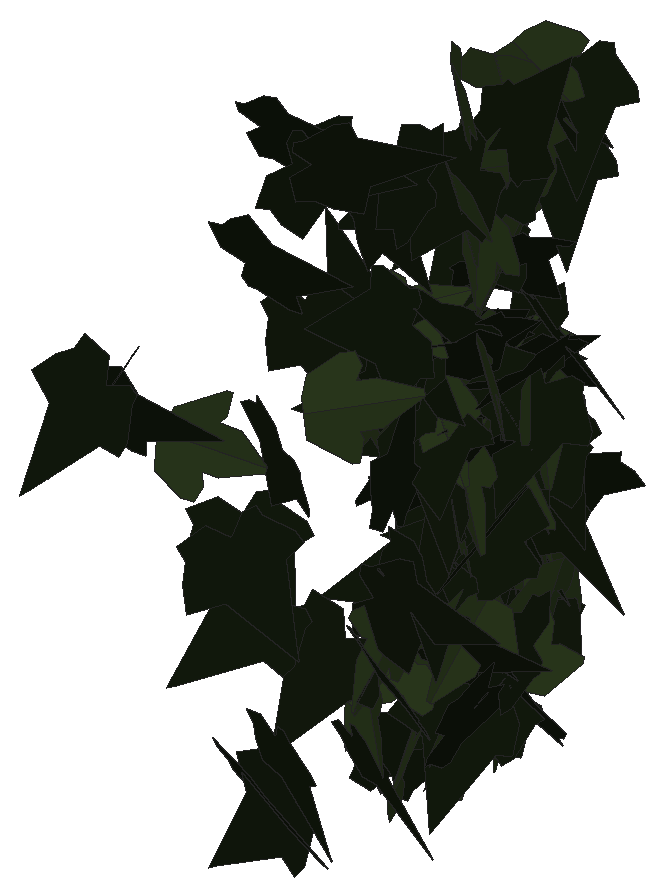
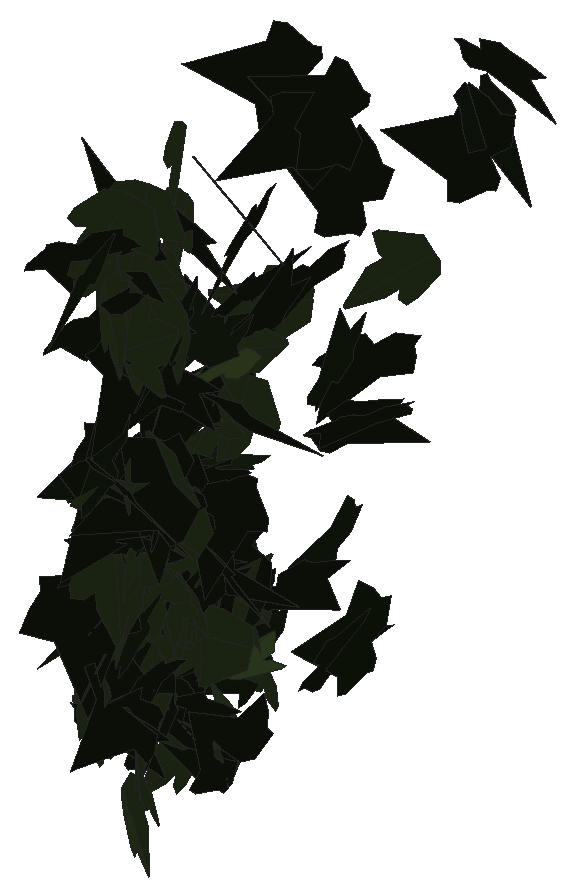
# SketchUp Ruby script. Lengths in inches.
U = 1.inch
M = Sketchup.active_model
def pt(a) = Geom::Point3d.new(a.map { |v| v * U })
def face(e, loops, mat)
  f = e.add_face(loops[0].map { |a| pt(a) })
  loops[1..].each { |l| e.add_face(l.map { |a| pt(a) }).erase! }
  f.material = f.back_material = mat if mat
  f
end
# faces: each face lists its corners as indices into pts; further lists are holes
def faces(e, pts, list, mat = nil) = list.each { |f| face(e, (f[0].is_a?(Array) ? f : [f]).map { |l| l.map { |i| pts[i] } }, mat) }
# xy, xz, yz: faces in a plane at the given z, y or x. An outline is a flat list of corners, or four numbers for a rectangle; further outlines are holes
def ring(l) = l.size == 4 ? [[l[0], l[1]], [l[2], l[1]], [l[2], l[3]], [l[0], l[3]]] : l.each_slice(2).to_a
def flat(e, list, mat, &to3) = list.each { |f| face(e, (f[0].is_a?(Array) ? f : [f]).map { |l| ring(l).map { |u, v| to3.(u, v) } }, mat) }
def xy(e, z, list, mat = nil) = flat(e, list, mat) { |x, y| [x, y, z] }
def xz(e, y, list, mat = nil) = flat(e, list, mat) { |x, z| [x, y, z] }
def yz(e, x, list, mat = nil) = flat(e, list, mat) { |y, z| [x, y, z] }
def lines(e, pts, list) = list.each { |a, b| e.add_line(pt(pts[a]), pt(pts[b])) }
# prism: a flat outline (further loops are holes) pulled along v
def prism(e, loops, v, mat = nil)
  f = face(e, loops, mat); d = Geom::Vector3d.new(v.map { |x| x * U })
  f.pushpull(f.normal.samedirection?(d) ? d.length : -d.length)
end
def box(e, o, s, mat = nil) = prism(e, [[o, [o[0] + s[0], o[1], o[2]], [o[0] + s[0], o[1] + s[1], o[2]], [o[0], o[1] + s[1], o[2]]]], [0, 0, s[2]], mat)
def at(x, y, z, deg = 0) = Geom::Transformation.translation(pt([x, y, z])) * Geom::Transformation.rotation(ORIGIN, Z_AXIS, deg.degrees)
def axes(o, x, y, z) = Geom::Transformation.new([*x, 0, *y, 0, *z, 0, *pt(o).to_a, 1])
def part(name) = M.definitions.add(name)
# library, detail: a bought-in or finely detailed component or shape, given as its bounding box
def library(name, o, s) = part(name).tap { |d| box(d.entities, o, s) }
def detail(e, o, s) = box(e.add_group.entities, o, s)
def put(e, d, t, mat = nil) = e.add_instance(d, t).tap { |i| i.material = mat if mat }
def group(e, t, mat = nil) = e.add_group.tap { |g| g.transformation = t; g.material = mat if mat }.entities
root = M.entities
M.materials.add("efeu1").color = [18, 25, 13]
M.materials.add("efeu2").color = [43, 57, 29]
c1 = part("ivyleaf_9")
p = [[1.54,2.16,1.25],[1.36,2.04,1.19],[-0.21,0.99,0.68],[-0.71,1.11,0.82],[-0.85,0.86,0.67],[-0.8,0.17,0.21],
  [-0.9,-0.01,0.1],[-0.67,-0.16,-0.02],[-0.08,-0.08,-0.05],[-0.03,-0.6,-0.4],[0.65,-0.88,-0.66],[0.83,-0.6,-0.49],
  [1.29,-0.42,-0.43],[1.8125,-0.07,-0.26],[1.21,0.44,0.15]]
faces(c1.entities,p,[[0,1,2,3,4,5,6,7,8,9,10,11,12,13,14]],"efeu1")
c2 = part("ivyleaf_10")
p = [[0,0.5,-0.03],[-0.0625,2.02,-0.43],[-0.19,2.01,-0.46],[-0.54,1.05,-0.29],[-0.52,0.625,-0.18],[-0.83,0.76,-0.28],
  [-1.16,0.64,-0.33],[-1.15,0.33,-0.24],[-0.77,-0.39,0.02],[-0.3,-0.51,0.16],[0.04,-0.48,0.23],[-0.02,2.01,-0.4375],
  [-0.06,2.01,-0.43],[0.04,-0.49,0.23],[0.67,-0.49,0.14],[1.38,0.36,-0.2],[1.375,0.51,-0.24],[0.81,0.65,-0.19],
  [0.62,0.59,-0.15],[0.6,1.09,-0.28],[0.5,1.23,-0.31]]
faces(c2.entities,p,[[0,1,2,3,4,5,6,7,8,9,10],[11,12,0,13,14,15,16,17,18,19,20]],"efeu2")
put(root,c1,axes([52.54,222,233.4],[-0.12743,-0.13778,0.46344],[0.30064,0.35276,0.18755],[-0.37865,0.32646,-0.00706]))
put(root,c1,axes([52.47,223.08,240.19],[0.37005,-0.22634,-0.24867],[-0.21472,0.1255,-0.43376],[0.25877,0.42781,-0.00432]))
put(root,c1,axes([52.57,223.91,235.06],[0.14272,0.35572,0.32109],[0.12597,0.29539,-0.38324],[-0.46234,0.19029,-0.0053]))
put(root,c1,axes([52.22,219.8,234.22],[0.374,-0.25873,0.2078],[0.17217,-0.11637,-0.45477],[0.28369,0.41173,0.00205]))
put(root,c1,axes([52.32,219.75,237.35],[0.0377,-0.46985,-0.16678],[0.17017,0.16934,-0.4386],[0.46864,-0.02369,0.17268]))
put(root,c1,axes([52.33,223.42,237.99],[0.39492,0.17488,0.25191],[0.21611,0.1327,-0.43091],[-0.21757,0.44923,0.02923]))
put(root,c2,axes([52.91,223.47,239.78],[-0.23646,0.11889,-0.42421],[-0.36386,0.21873,0.26412],[0.24838,0.43361,-0.01693]))
put(root,c1,axes([52.625,221.02,235.4],[-0.25003,-0.4141,0.12651],[-0.06772,-0.10689,-0.48372],[0.42767,-0.25902,-0.00264]))
put(root,c2,axes([52.43,223.35,240.21],[-0.3398,0.20353,-0.30514],[0.24386,-0.18535,-0.39519],[-0.27399,-0.4174,0.0267]))
put(root,c1,axes([53,221.84,238.15],[-0.4116,0.12746,0.25365],[-0.26788,-0.02654,-0.42135],[-0.09394,-0.48275,0.09013]))
put(root,c2,axes([52.63,222.03,234.64],[-0.47623,-0.02563,0.15016],[0.06941,-0.47525,0.13899],[0.1356,0.15323,0.45622]))
put(root,c1,axes([52.21,220.25,241.83],[0.28379,0.17344,-0.37334],[0.32837,0.1781,0.33235],[0.24827,-0.43382,-0.01282]))
put(root,c2,axes([52.64,223.34,234.63],[-0.09644,0.44196,0.213],[-0.07762,0.2006,-0.45137],[-0.48443,-0.12013,0.02992]))
put(root,c2,axes([52.62,223.97,233.59],[0.22192,-0.44085,0.08005],[0.04515,-0.06687,-0.49345],[0.44577,0.22624,0.01013]))
put(root,c1,axes([52.82,216.8,240.35],[-0.28664,0.37913,-0.15524],[0.09516,-0.12267,-0.47529],[-0.39847,-0.30202,-0.00183]))
put(root,c1,axes([52.75,223.39,239.44],[-0.45151,-0.2066,-0.05876],[0.06151,0.00669,-0.49616],[0.2058,-0.45527,0.01937]))
put(root,c1,axes([52.73,221.97,237.1875],[0.1117,0.48678,0.02385],[0.00703,0.02286,-0.49943],[-0.48731,0.11191,-0.00174]))
put(root,c2,axes([52.51,223.09,236.35],[0.4207,-0.21305,0.16621],[0.15861,-0.05428,-0.47106],[0.21876,0.44907,0.02191]))
put(root,c2,axes([52.79,223.36,236.97],[0.07256,0.12483,0.4787],[-0.25109,0.42616,-0.07307],[-0.42625,-0.22979,0.12453]))
put(root,c1,axes([52.83,223.27,237.96],[-0.03612,0.49855,0.01178],[-0.00711,0.01129,-0.49982],[-0.49864,-0.03628,0.00627]))
put(root,c2,axes([52.38,223.24,237.09],[-0.20906,-0.1301,0.43517],[0.37201,0.22579,0.24622],[-0.26058,0.42672,0.00239]))
put(root,c1,axes([52.6875,220.09,233.875],[-0.14326,-0.29748,0.37548],[-0.13764,-0.34982,-0.32967],[0.45884,-0.19782,0.01834]))
put(root,c1,axes([52.8125,221.21,239.09],[-0.15478,-0.41276,0.23595],[0.10415,0.21268,0.44036],[-0.46389,0.18547,0.02014]))
put(root,c1,axes([52.47,220.1875,238.04],[-0.00705,-0.27387,0.41827],[0.11007,-0.40889,-0.26588],[0.48768,0.08833,0.06605]))
put(root,c2,axes([52.51,218.49,238.91],[0.08143,0.20329,0.44949],[0.16024,0.41997,-0.21897],[-0.46658,0.17971,0.00324]))
put(root,c2,axes([52.91,223.1,236.1],[-0.45999,0.01901,0.19505],[-0.19532,-0.08516,-0.45233],[0.01602,-0.49233,0.08577]))
put(root,c2,axes([52.36,223.39,238.02],[0.26856,0.00029,0.42175],[0.42173,0.00518,-0.26855],[-0.00452,0.49997,0.00254]))
put(root,c2,axes([52.88,221.66,233.48],[0.1955,-0.08855,0.4516],[-0.28684,0.36024,0.19481],[-0.35987,-0.33524,0.09006]))
put(root,c2,axes([52.52,223.88,234.04],[0.3234,-0.23048,0.30379],[0.26475,-0.15097,-0.39638],[0.27444,0.41724,0.0244]))
put(root,c1,axes([52.5625,220.53,239.68],[0.13999,-0.42507,-0.22297],[-0.04554,0.21945,-0.44695],[0.47784,0.14545,0.02273]))
put(root,c2,axes([52.77,222.9,235.9],[-0.41577,0.27742,0.01329],[-0.01509,0.00132,-0.49977],[-0.27733,-0.41598,0.00728]))
put(root,c2,axes([52.61,221.97,239.01],[0.43239,-0.13329,-0.21278],[0.16186,0.4719,0.0333],[0.19195,-0.09768,0.45124]))
put(root,c2,axes([52.875,223.98,236.92],[-0.38979,-0.30826,0.05513],[-0.04397,-0.03327,-0.49695],[0.31005,-0.39226,-0.00118]))
put(root,c1,axes([52.99,222.25,236.43],[-0.49114,0.08693,-0.03502],[0.03433,-0.00701,-0.49877],[-0.08721,-0.49233,0.00092]))
put(root,c1,axes([52.35,219.81,240.44],[0.18372,-0.12807,0.44704],[0.40533,-0.1915,-0.22144],[0.22794,0.44376,0.03345]))
put(root,c2,axes([52.42,222.25,235.1875],[0.11033,-0.00862,-0.4876],[0.46689,0.14627,0.10306],[0.14087,-0.47805,0.04032]))
put(root,c2,axes([52.83,221.66,238.97],[-0.09962,0.18434,-0.45398],[-0.13483,-0.45569,-0.15545],[-0.47106,0.09145,0.1405]))
put(root,c1,axes([52.84,222.84,235.66],[-0.11595,-0.21492,0.43631],[-0.21428,-0.38009,-0.24417],[0.43662,-0.24361,-0.00396]))
put(root,c1,axes([53.12,222.23,236.02],[-0.42038,-0.04415,0.26707],[-0.26448,-0.03811,-0.42261],[0.05767,-0.49659,0.00869]))
put(root,c1,axes([52.66,223.93,235.15],[-0.03109,-0.49497,0.06354],[-0.01283,-0.06285,-0.49587],[0.49887,-0.03246,-0.00879]))
put(root,c1,axes([53.125,223.87,238],[-0.45371,0.17036,0.123],[-0.1198,0.03073,-0.48446],[-0.17262,-0.46908,0.01293]))
put(root,c2,axes([52.86,223.42,238.02],[0.0425,-0.49817,-0.00431],[-0.00458,0.00394,-0.49996],[0.49817,0.04254,-0.00422]))
put(root,c1,axes([52.6,223.73,236.08],[0.38289,-0.31099,-0.08171],[-0.06145,0.05394,-0.49327],[0.31562,0.38778,0.00309]))
put(root,c2,axes([52.84,221.46,238.21],[-0.09418,-0.41566,-0.26146],[0.06945,0.25227,-0.42607],[0.48611,-0.11657,0.01022]))
put(root,c1,axes([52.57,222.9,237.42],[0.37894,0.12388,0.30176],[0.24718,0.19277,-0.38954],[-0.21285,0.44441,0.08485]))
put(root,c2,axes([52.68,222.33,235.25],[0.018,-0.17464,-0.46816],[0.2738,0.39532,-0.13695],[0.41798,-0.25143,0.10986]))
put(root,c1,axes([52.76,221.38,240.76],[0.27369,-0.27786,-0.31287],[-0.21444,0.22789,-0.38997],[0.35932,0.34765,0.00557]))
put(root,c1,axes([52.7,220.19,241.58],[0.07228,0.06448,-0.49053],[-0.03702,0.49505,0.05962],[0.49336,0.0277,0.07634]))
put(root,c1,axes([52.4375,217.19,239.88],[0.28667,-0.06983,0.40366],[0.3897,-0.10543,-0.29499],[0.12631,0.48374,-0.00602]))
put(root,c2,axes([52.79,223.56,236.57],[0.4657,0.18166,-0.01117],[-0.00989,-0.00538,-0.49987],[-0.18174,0.4658,-0.00142]))
put(root,c1,axes([52.79,223.39,237.56],[0.42579,-0.08179,-0.24902],[-0.23767,0.07984,-0.4326],[0.11052,0.48676,0.02911]))
put(root,c2,axes([53.03,222.99,236.19],[-0.2906,-0.32651,0.24279],[-0.11953,-0.21668,-0.43447],[0.38893,-0.31055,0.04788]))
put(root,c2,axes([52.6,221.42,234.52],[0.30034,-0.14463,0.37266],[0.35553,-0.11644,-0.33172],[0.18274,0.46424,0.0329]))
put(root,c2,axes([52.93,223.89,235.47],[-0.07918,0.49287,0.02846],[-0.08407,0.01494,-0.49266],[-0.48648,-0.08281,0.0805]))
put(root,c2,axes([52.79,223.78,237.8125],[0.24713,0.40604,0.1551],[0.0681,0.14004,-0.47513],[-0.42929,0.25597,0.01391]))
put(root,c2,axes([52.87,221.61,235.4],[-0.04538,-0.30078,0.39682],[0.14398,-0.38937,-0.27867],[0.47667,0.08898,0.12195]))
put(root,c1,axes([53.08,219.3,236.78],[-0.34226,-0.2941,0.21533],[-0.15663,-0.14805,-0.45116],[0.32913,-0.37628,0.00921]))
put(root,c1,axes([52.86,221.6,238.81],[0.16506,-0.21205,-0.42165],[-0.20934,0.36746,-0.26674],[0.423,0.26459,0.03253]))
put(root,c1,axes([52.92,223.95,237.06],[-0.3232,-0.37439,-0.07332],[0.05656,0.04801,-0.49447],[0.37728,-0.32792,0.01131]))
put(root,c1,axes([53.04,223.97,234.71],[-0.45814,-0.18174,-0.08415],[0.08637,0.01028,-0.49238],[0.1807,-0.46569,0.02198]))
put(root,c2,axes([53.15,224.19,235.08],[0.25927,-0.11087,-0.4129],[-0.25229,0.35017,-0.25244],[0.34515,0.33924,0.12564]))
put(root,c1,axes([52.81,223.5,236.59],[0.39833,-0.2769,-0.12106],[0.09584,-0.0742,0.48509],[-0.28661,-0.40966,-0.00603]))
put(root,c1,axes([53.13,216.33,240.72],[-0.48736,-0.09764,-0.05426],[0.05338,0.00979,-0.49705],[0.09813,-0.49028,0.00088]))
put(root,c2,axes([52.93,223.8,236.14],[-0.34201,0.34766,-0.11026],[0.06761,-0.0881,-0.48751],[-0.35841,-0.34838,0.01325]))
put(root,c1,axes([52.93,223.62,237.78],[0.2958,0.37907,0.13715],[0.065,0.12303,-0.48025],[-0.39784,0.30194,0.0235]))
put(root,c1,axes([52.68,223.44,234.32],[0.11825,-0.25127,0.41579],[0.19304,-0.3684,-0.27753],[0.44582,0.22616,0.00988]))
put(root,c2,axes([53.19,222.47,235.54],[-0.15909,-0.25945,0.39671],[-0.16932,-0.35974,-0.30318],[0.44274,-0.23081,0.0266]))
put(root,c2,axes([52.97,222.95,235.46],[-0.20052,0.4577,-0.01735],[0.00964,-0.01472,-0.49969],[-0.45793,-0.20074,-0.00292]))
put(root,c2,axes([53.04,222.32,233.63],[0.05784,0.11816,0.48238],[-0.12938,0.47246,-0.10022],[-0.47949,-0.11323,0.08523]))
put(root,c1,axes([52.91,222.46,237.37],[-0.08067,-0.48674,-0.08109],[0.03533,0.07626,-0.49289],[0.49218,-0.08525,0.02209]))
put(root,c1,axes([53.17,222.26,237.14],[0.052,0.4968,-0.02213],[-0.00281,-0.02196,-0.49951],[-0.49728,0.05208,0.00051]))
put(root,c2,axes([52.85,222.26,237.93],[-0.12365,-0.48419,0.01654],[0.34608,-0.10022,-0.34668],[0.33903,-0.07429,0.35991]))
put(root,c1,axes([53.29,222.9375,240.0625],[-0.48694,0.10081,-0.05224],[-0.05099,0.01138,0.49726],[0.10144,0.4896,-0.0008]))
put(root,c2,axes([53.11,223.15,241.57],[-0.49374,-0.07449,-0.02586],[0.02587,0.00188,-0.49933],[0.07448,-0.49442,0.002]))
put(root,c1,axes([52.81,222.25,237.61],[-0.12369,-0.48261,-0.04229],[0.34495,-0.05709,-0.35743],[0.34017,-0.11759,0.34707]))
put(root,c1,axes([53.38,222.97,234.1875],[-0.45839,-0.06228,0.18973],[-0.18551,-0.04299,-0.46232],[0.0739,-0.49424,0.01631]))
put(root,c1,axes([53.4,221.43,241.1],[-0.43341,0.23508,0.08301],[-0.07225,0.04091,-0.49306],[-0.23861,-0.43939,-0.00149]))
put(root,c2,axes([53.1,223.77,240.44],[0.15336,-0.47556,0.01794],[0.04804,-0.00328,-0.49768],[0.47347,0.15437,0.04468]))
put(root,c2,axes([53.18,223.13,240.27],[-0.12397,-0.47931,0.06991],[-0.00348,-0.07128,-0.49488],[0.48437,-0.12319,0.01434]))
put(root,c1,axes([52.9375,218.81,237.69],[0.01597,-0.35968,-0.34695],[0.04142,0.34688,-0.35771],[0.49803,-0.01732,0.04087]))
put(root,c1,axes([53.17,221.45,239.25],[0.09895,-0.39931,-0.28419],[0.07481,-0.27422,0.41135],[-0.48437,-0.12392,0.00548]))
put(root,c1,axes([53.22,224.1,236.35],[0.19902,0.41279,-0.19999],[-0.08718,-0.17998,-0.45826],[-0.45032,0.21728,0.00033]))
put(root,c1,axes([53.09,222.98,239.35],[0.29745,0.39529,0.07257],[0.03843,0.0619,-0.49466],[-0.40006,0.29986,0.00645]))
put(root,c2,axes([53.08,222.48,236.59],[-0.19813,0.45382,-0.0692],[0.03352,-0.06087,-0.49515],[-0.45784,-0.20085,-0.0063]))
put(root,c1,axes([53.13,222.62,234.15],[-0.29483,-0.39976,-0.05717],[0.03199,0.04744,-0.49672],[0.40256,-0.29655,-0.0024]))
put(root,c1,axes([53.2,222.31,238.67],[0.17342,0.4686,0.01835],[0.00566,0.01748,-0.49966],[-0.46893,0.17351,0.00075]))
put(root,c1,axes([53.32,223.73,236.93],[-0.45857,-0.19751,0.02654],[-0.02468,-0.00979,-0.49929],[0.19775,-0.45923,-0.00077]))
put(root,c2,axes([53.27,222.21,241.93],[-0.34345,0.34466,0.11512],[-0.11413,0.04808,-0.48442],[-0.34499,-0.35903,0.04565]))
put(root,c1,axes([53.04,223.89,237],[0.08696,-0.44568,-0.2093],[-0.02934,0.20747,-0.45398],[0.4915,0.09124,0.00993]))
put(root,c1,axes([52.92,220.92,234.32],[0.38366,-0.3181,0.04024],[0.03431,-0.02166,-0.49835],[0.31879,0.38515,0.00521]))
put(root,c1,axes([52.98,221.33,234.97],[0.41462,-0.20985,-0.18455],[0.16969,-0.07329,0.46458],[-0.22203,-0.44788,0.01044]))
put(root,c1,axes([53.17,223.85,241.27],[0.36383,-0.10276,-0.32721],[-0.27779,0.19147,-0.36901],[0.20114,0.45031,0.08223]))
put(root,c1,axes([53.4,222.54,234.32],[-0.24916,0.37011,-0.22569],[0.095,-0.20737,-0.44494],[-0.42296,-0.2646,0.03302]))
put(root,c2,axes([53.2,223.16,239.62],[0.13511,-0.40286,0.26353],[0.08717,-0.24871,-0.4249],[0.47344,0.16077,0.00303]))
put(root,c1,axes([53.38,223.18,238.01],[0.00239,0.49957,-0.02069],[-0.00125,-0.02069,-0.49957],[-0.49999,0.00244,0.00115]))
put(root,c2,axes([53.18,223.375,234.3],[0.49569,0.06457,-0.0109],[0.00991,0.00826,0.49983],[0.06473,-0.49574,0.00691]))
put(root,c1,axes([52.98,222.26,239.09],[-0.12573,-0.4049,0.26504],[0.35039,-0.26505,-0.2387],[0.33379,0.12571,0.3504]))
put(root,c1,axes([53.01,221.98,235.98],[0.07386,-0.45049,0.20398],[0.0877,-0.19104,-0.45367],[0.48667,0.1028,0.0508]))
put(root,c2,axes([53.12,223.55,241.61],[-0.28247,-0.29732,-0.28603],[0.25731,0.144,-0.4038],[0.32249,-0.37532,0.07166]))
put(root,c1,axes([53.625,222.77,236.22],[-0.351,0.05189,0.35228],[-0.34983,-0.14252,-0.32757],[0.06642,-0.47644,0.13636]))
put(root,c2,axes([53.1875,223.08,236.55],[0.49696,0.04569,0.03071],[0.02709,0.03985,-0.49767],[-0.04792,0.49631,0.03713]))
put(root,c2,axes([53.35,223.33,240.75],[-0.29703,-0.40118,-0.0287],[0.02144,0.01984,-0.49915],[0.40164,-0.29775,0.00542]))
put(root,c1,axes([53.14,224.12,240.38],[-0.02055,-0.49752,-0.04525],[0.01005,0.04487,-0.49788],[0.49948,-0.02137,0.00815]))
put(root,c1,axes([53.5,222.2,240.89],[-0.49784,0.00252,-0.0464],[0.04645,0.01513,-0.49761],[-0.0011,-0.49976,-0.01529]))
put(root,c1,axes([53.35,220.99,237.36],[-0.00322,-0.24186,0.4376],[0.15989,0.41413,0.23007],[-0.47374,0.14141,0.07468]))
put(root,c2,axes([53.15,222.47,237.11],[-0.32191,0.13535,-0.35784],[0.22047,-0.31658,-0.31807],[-0.31268,-0.36257,0.14414]))
put(root,c1,axes([53.01,223.92,238.31],[0.40188,-0.28471,0.08619],[0.0742,-0.04436,-0.49247],[0.28807,0.40862,0.0066]))
put(root,c1,axes([53.52,222.23,236.39],[-0.07586,0.4699,0.1531],[-0.01819,0.15213,-0.47595],[-0.49388,-0.07778,-0.00599]))
put(root,c1,axes([53.0625,219.39,235.06],[0.29037,-0.38661,0.12734],[0.06826,-0.10796,-0.48341],[0.40128,0.29812,-0.00992]))
put(root,c2,axes([53.4,223.65,235.32],[0.03754,-0.48964,0.09402],[0.02024,-0.09271,-0.49091],[0.49818,0.04067,0.01286]))
put(root,c1,axes([52.97,221.22,235.95],[0.22038,0.03633,-0.44734],[0.33824,0.31412,0.19214],[0.295,-0.38731,0.11387]))
put(root,c1,axes([53.71,222.84,234.93],[-0.42358,0.24655,0.09895],[-0.08608,0.0488,-0.49011],[-0.25133,-0.43224,0.0011]))
put(root,c2,axes([53.35,222.52,238.55],[-0.31777,0.38033,-0.06612],[0.04017,-0.0526,-0.4956],[-0.38394,-0.32028,0.00287]))
put(root,c2,axes([53.5,222.32,240.22],[-0.47759,0.13541,0.05976],[-0.08819,-0.09819,-0.48227],[-0.11887,-0.47119,0.11768]))
put(root,c2,axes([53.43,222.34,235.4],[0.16507,0.35159,-0.31486],[-0.14672,-0.27881,-0.38825],[-0.44858,0.22057,0.01112]))
put(root,c1,axes([52.98,222.09,235.07],[0.27142,-0.10182,0.40739],[0.39831,-0.09118,-0.28816],[0.13297,0.48096,0.03161]))
put(root,c2,axes([53.47,221.96,240.79],[-0.42549,0.25352,0.06846],[-0.05872,0.03519,-0.49529],[-0.25595,-0.42952,-0.00017]))
put(root,c1,axes([53.17,223.82,236.09],[0.33078,-0.36164,-0.09902],[-0.00982,0.12364,-0.48437],[0.37482,0.32238,0.07469]))
put(root,c1,axes([53.34,223.16,233.99],[0.43967,-0.23314,0.04832],[-0.04106,0.02571,0.49765],[-0.23453,-0.44157,0.00347]))
put(root,c2,axes([53.39,223.45,237.59],[-0.04489,0.49395,-0.06325],[-0.00018,-0.06352,-0.49595],[-0.49798,-0.0445,0.00588]))
put(root,c1,axes([53.33,224.125,241.32],[-0.15207,-0.45476,-0.14167],[0.07652,0.12346,-0.47844],[0.47013,-0.16719,0.03205]))
put(root,c1,axes([53.45,223.39,237.73],[-0.26552,-0.42349,-0.01255],[0.00546,0.01139,-0.49984],[0.42364,-0.26557,-0.00142]))
put(root,c2,axes([53.18,220.1,238.85],[0.07795,-0.02179,-0.4934],[0.43313,0.24305,0.0577],[0.23733,-0.43641,0.05677]))
put(root,c1,axes([53.51,221.72,234.31],[0.096,0.27608,0.40567],[0.16167,0.37248,-0.29175],[-0.4633,0.18719,-0.01775]))
put(root,c1,axes([53.22,219.88,241.9],[0.1852,0.25712,-0.38677],[0.16371,0.35351,0.31341],[0.43462,-0.24273,0.04676]))
put(root,c1,axes([53.375,222.93,240.87],[-0.21176,0.20557,0.40361],[0.28632,-0.28448,0.29511],[0.35097,0.35611,0.00277]))
